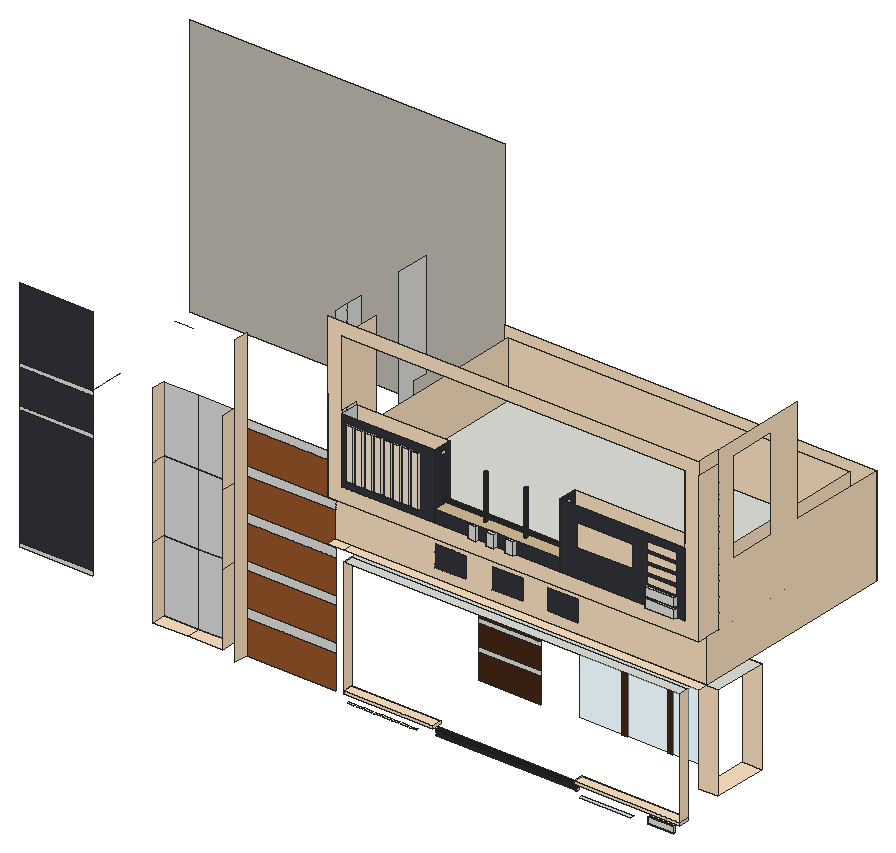
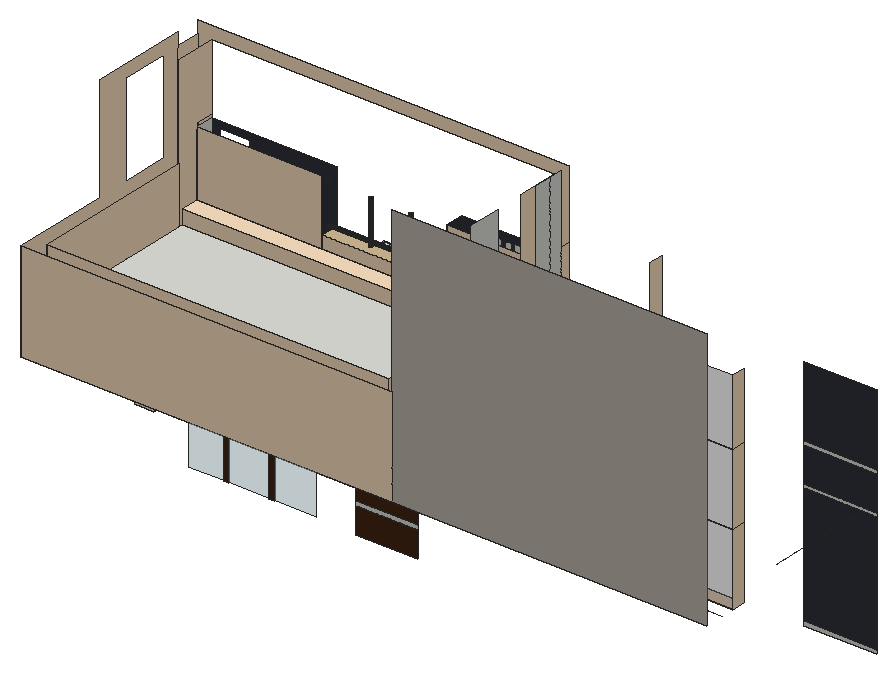
# SketchUp Ruby script. Lengths in inches.
U = 1.inch
M = Sketchup.active_model
def pt(a) = Geom::Point3d.new(a.map { |v| v * U })
def face(e, loops, mat)
  f = e.add_face(loops[0].map { |a| pt(a) })
  loops[1..].each { |l| e.add_face(l.map { |a| pt(a) }).erase! }
  f.material = f.back_material = mat if mat
  f
end
# faces: each face lists its corners as indices into pts; further lists are holes
def faces(e, pts, list, mat = nil) = list.each { |f| face(e, (f[0].is_a?(Array) ? f : [f]).map { |l| l.map { |i| pts[i] } }, mat) }
# xy, xz, yz: faces in a plane at the given z, y or x. An outline is a flat list of corners, or four numbers for a rectangle; further outlines are holes
def ring(l) = l.size == 4 ? [[l[0], l[1]], [l[2], l[1]], [l[2], l[3]], [l[0], l[3]]] : l.each_slice(2).to_a
def flat(e, list, mat, &to3) = list.each { |f| face(e, (f[0].is_a?(Array) ? f : [f]).map { |l| ring(l).map { |u, v| to3.(u, v) } }, mat) }
def xy(e, z, list, mat = nil) = flat(e, list, mat) { |x, y| [x, y, z] }
def xz(e, y, list, mat = nil) = flat(e, list, mat) { |x, z| [x, y, z] }
def yz(e, x, list, mat = nil) = flat(e, list, mat) { |y, z| [x, y, z] }
def lines(e, pts, list) = list.each { |a, b| e.add_line(pt(pts[a]), pt(pts[b])) }
# prism: a flat outline (further loops are holes) pulled along v
def prism(e, loops, v, mat = nil)
  f = face(e, loops, mat); d = Geom::Vector3d.new(v.map { |x| x * U })
  f.pushpull(f.normal.samedirection?(d) ? d.length : -d.length)
end
def box(e, o, s, mat = nil) = prism(e, [[o, [o[0] + s[0], o[1], o[2]], [o[0] + s[0], o[1] + s[1], o[2]], [o[0], o[1] + s[1], o[2]]]], [0, 0, s[2]], mat)
def at(x, y, z, deg = 0) = Geom::Transformation.translation(pt([x, y, z])) * Geom::Transformation.rotation(ORIGIN, Z_AXIS, deg.degrees)
def axes(o, x, y, z) = Geom::Transformation.new([*x, 0, *y, 0, *z, 0, *pt(o).to_a, 1])
def part(name) = M.definitions.add(name)
# library, detail: a bought-in or finely detailed component or shape, given as its bounding box
def library(name, o, s) = part(name).tap { |d| box(d.entities, o, s) }
def detail(e, o, s) = box(e.add_group.entities, o, s)
def put(e, d, t, mat = nil) = e.add_instance(d, t).tap { |i| i.material = mat if mat }
def group(e, t, mat = nil) = e.add_group.tap { |g| g.transformation = t; g.material = mat if mat }.entities
root = M.entities
M.materials.add("[0012_Bisque]").color = [255, 228, 196]
M.materials.add("[0028_AntiqueWhite]").color = [250, 235, 215]
M.materials.add("[Color M08]").color = [30, 30, 30]
M.materials.add("[Color M09]").color = [0, 0, 0]
M.materials.add("[Field Rectangle Tile]").color = [196, 189, 179]
M.materials.add("[Formica Beige]").color = [211, 187, 149]
M.materials.add("[Formica Laminate Dark]").color = [50, 53, 60]
M.materials.add("[Translucent Glass Gray]").color = [128, 128, 128]
M.materials["[Translucent Glass Gray]"].alpha = 0.5
M.materials.add("[Translucent Glass Safety]").color = [204, 235, 244]
M.materials["[Translucent Glass Safety]"].alpha = 0.5
M.materials.add("[Wood Cherry Original]").color = [152, 86, 42]
M.materials.add("[Wood Veneer 01]").color = [68, 40, 21]
box(root,[409.26,39.8,166.78],[15.5,0.87,3.19])
xy(root,166.28,[[409.2,39.8,424.7,40.67]])
xy(root,166.58,[[368.61,38.8,399.74,40.67]])
xy(root,168.02,[[227.93,39.48,232.05,40.67],[233.37,39.48,237.49,40.67],[238.43,39.48,242.55,40.67],[244.05,39.48,248.18,40.67],[249.43,39.48,253.55,40.67],
  [254.74,39.48,258.87,40.67],[260.12,39.48,264.24,40.67],[265.49,39.48,269.62,40.67]],"[0028_AntiqueWhite]")
xy(root,168.7,[[[278.51,42.95,363.63,45.58],[336.54,43.14,336.79,43.17,337.04,43.27,337.24,43.43,337.4,43.64,337.5,43.88,337.54,44.14,337.5,44.4,337.4,44.64,337.24,44.85,337.04,45.01,336.79,45.11,336.54,45.14,336.28,45.11,336.04,45.01,335.83,44.85,335.67,44.64,335.57,44.4,335.54,44.14,335.57,43.88,335.67,43.64,335.83,43.43,336.04,43.27,336.28,43.17]]],"[Color M08]")
xy(root,168.8125,[[305.54,43.14,305.79,43.17,306.04,43.27,306.24,43.43,306.4,43.64,306.5,43.88,306.54,44.14,306.5,44.4,306.4,44.64,306.24,44.85,306.04,45.01,305.79,45.11,305.54,45.14,305.28,45.11,305.04,45.01,304.83,44.85,304.67,44.64,304.57,44.4,304.54,44.14,304.57,43.88,304.67,43.64,304.83,43.43,305.04,43.27,305.28,43.17]])
xy(root,170.07,[[278.51,42.95,363.63,45.58]],"[Color M08]")
xy(root,171.14,[[111.55,38.36,132.61,46.73],[132.61,38.36,153.67,46.73]],"[0012_Bisque]")
xy(root,171.25,[[224.52,40.67,278.51,46.73],[363.63,40.67,427.75,46.73]])
xy(root,173,[[224.52,40.67,278.51,46.73],[363.63,40.67,427.75,46.73]],"[0012_Bisque]")
xy(root,185.0625,[[427.75,54.79,439.21,87.8]],"[0012_Bisque]")
xy(root,242.43,[[224.52,40.67,427.75,46.73],[224.52,46.73,427.75,54.79],[427.75,54.79,439.21,87.8]])
xy(root,249,[[215,46.73,215,162.99,224.52,162.99,224.52,54.79,427.75,54.79,427.75,63.87,439.21,63.87,439.21,46.73],[224.52,54.79,427.75,96.17],[427.75,63.87,439.21,96.36],[224.52,96.17,427.75,107.95],[427.75,96.36,439.21,105.43],
  [427.75,105.43,439.21,174.44],[224.52,107.95,427.75,162.99],[215,162.99,224.52,174.44],[224.52,162.99,427.75,174.44]])
xy(root,249,[[215,40.67,224.52,46.73],[224.52,40.67,439.21,46.73]],"[0012_Bisque]")
xy(root,274.6875,[[215,40.67,223.75,46.73],[223.75,40.67,430.46,46.73],[430.46,40.67,439.21,46.73],[215,46.73,223.75,55.48],[223.75,46.73,430.46,55.48],
  [430.46,46.73,439.21,55.48],[215,55.48,223.75,65.9],[223.75,63.28,430.46,165.7],[215,94.79,223.75,105.21]])
xy(root,283.0625,[[301.05,38.8,305.76,40.67],[312.17,38.8,316.88,40.67],[323.67,38.8,328.38,40.67],[407.7,39.05,425.58,40.67],[223.75,40.67,279.65,51.97],
  [279.65,40.67,355.06,51.97],[355.06,40.67,430.46,51.97]])
xy(root,283.0625,[[223.75,51.97,430.46,63.28]],"[0012_Bisque]")
xy(root,287.67,[[227.14,39.36,231.39,40.67],[232.64,39.36,236.89,40.67],[238.51,39.36,242.76,40.67],[244.08,39.36,248.33,40.67],[249.76,39.36,254.01,40.67],
  [255.33,39.36,259.58,40.67],[260.95,39.36,265.2,40.67],[266.39,39.36,270.64,40.67]])
xy(root,288.0625,[[407.7,39.05,425.58,40.67]])
xy(root,289.37,[[407.7,39.05,425.58,40.67]])
xy(root,290.6875,[[301.05,38.8,305.76,40.67],[312.17,38.8,316.88,40.67],[323.67,38.8,328.38,40.67],[305.63,45.65,305.4,45.68,305.19,45.77,305.01,45.91,304.87,46.09,304.78,46.3,304.75,46.53,304.78,46.75,304.87,46.96,305.01,47.15,305.19,47.29,305.4,47.37,305.63,47.4,305.85,47.37,306.07,47.29,306.25,47.15,306.39,46.96,306.47,46.75,306.5,46.53,306.47,46.3,306.39,46.09,306.25,45.91,306.07,45.77,305.85,45.68],[330.07,45.65,329.84,45.68,329.63,45.77,329.45,45.91,329.31,46.09,329.22,46.3,329.19,46.53,329.22,46.75,329.31,46.96,329.45,47.15,329.63,47.29,329.84,47.37,330.07,47.4,330.29,47.37,330.5,47.29,330.68,47.15,330.82,46.96,330.91,46.75,330.94,46.53,330.91,46.3,330.82,46.09,330.68,45.91,330.5,45.77,330.29,45.68]])
xy(root,290.6875,[[[279.65,40.67,355.06,51.97],[330.07,45.65,329.84,45.68,329.63,45.77,329.45,45.91,329.31,46.09,329.22,46.3,329.19,46.53,329.22,46.75,329.31,46.96,329.45,47.15,329.63,47.29,329.84,47.37,330.07,47.4,330.29,47.37,330.5,47.29,330.68,47.15,330.82,46.96,330.91,46.75,330.94,46.53,330.91,46.3,330.82,46.09,330.68,45.91,330.5,45.77,330.29,45.68],[305.63,45.65,305.4,45.68,305.19,45.77,305.01,45.91,304.87,46.09,304.78,46.3,304.75,46.53,304.78,46.75,304.87,46.96,305.01,47.15,305.19,47.29,305.4,47.37,305.63,47.4,305.85,47.37,306.07,47.29,306.25,47.15,306.39,46.96,306.47,46.75,306.5,46.53,306.47,46.3,306.39,46.09,306.25,45.91,306.07,45.77,305.85,45.68]]],"[Formica Beige]")
xy(root,294.37,[[407.7,39.05,425.58,40.67]])
xz(root,38.8,[[301.05,283.0625,305.76,290.6875],[312.17,283.0625,316.88,290.6875],[323.67,283.0625,328.38,290.6875]])
xz(root,39.05,[[407.7,283.0625,425.58,288.0625],[407.7,289.37,425.58,294.37]])
xz(root,39.36,[[227.14,287.67,231.39,317.98],[232.64,287.67,236.89,317.98],[238.51,287.67,242.76,317.98],[244.08,287.67,248.33,317.98],[249.76,287.67,254.01,317.98],
  [255.33,287.67,259.58,317.98],[260.95,287.67,265.2,317.98],[266.39,287.67,270.64,317.98]],"[0028_AntiqueWhite]")
xz(root,40.67,[[301.05,283.0625,305.76,290.6875],[312.17,283.0625,316.88,290.6875],[323.67,283.0625,328.38,290.6875],[407.7,283.0625,425.58,288.0625],[227.14,287.67,231.39,317.98],
  [232.64,287.67,236.89,317.98],[238.51,287.67,242.76,317.98],[244.08,287.67,248.33,317.98],[249.76,287.67,254.01,317.98],[255.33,287.67,259.58,317.98],
  [260.95,287.67,265.2,317.98],[266.39,287.67,270.64,317.98],[407.7,289.37,425.58,294.37]])
xz(root,40.67,[[224.52,171.25,278.51,173],[363.63,171.25,427.75,173],[215,274.6875,439.21,274.6875,439.21,364.53,430.46,364.53,430.46,283.0625,223.75,283.0625,223.75,364.53,439.21,364.53,439.21,372.25,215,372.25]],"[0012_Bisque]")
xz(root,40.67,[[[223.75,283.0625,279.65,322.3125],[227.14,287.67,231.39,317.98],[232.64,287.67,236.89,317.98],[238.51,287.67,242.76,317.98],[244.08,287.67,248.33,317.98],[249.76,287.67,254.01,317.98],[255.33,287.67,259.58,317.98],[260.95,287.67,265.2,317.98],[266.39,287.67,270.64,317.98]],[279.65,283.0625,301.05,290.6875],[305.76,283.0625,312.17,290.6875],[316.88,283.0625,323.67,290.6875],[328.38,283.0625,355.06,290.6875],
  [[355.06,283.0625,407.7,283.0625,407.7,288.0625,425.58,288.0625,425.58,283.0625,430.46,283.0625,430.46,322.3125,355.06,322.3125],[365.58,300,398.96,313.68],[407.7,313.43,425.58,318.43],[407.7,307.12,425.58,312.12],[407.7,301.12,425.58,306.12],[407.7,294.93,425.58,299.93],[407.7,289.37,425.58,294.37]]],"[Formica Laminate Dark]")
xz(root,42.95,[[278.51,168.7,363.63,170.07]],"[Color M08]")
xz(root,45.58,[[278.51,168.7,363.63,170.07]],"[Color M08]")
xz(root,46.73,[[24.6875,177.73,68.38,180.02],[161.14,187.61,215,192.76],[161.14,213.23,215,218.39],[161.14,238.86,215,244.01],[24.6875,251.85,68.38,254.15],
  [161.14,264.48,215,269.64],[24.6875,275.16,68.38,277.46],[161.14,290.11,215,295.26]])
xz(root,46.73,[[224.52,171.25,278.51,173],[363.63,171.25,427.75,173],[[215,249,439.21,274.6875],[275.14,254.7,294.2,267.83],[309.26,254.7,328.33,267.83],[342.45,254.7,361.51,267.83]]],"[0012_Bisque]")
xz(root,46.73,[[24.6875,180.02,68.38,251.85],[24.6875,254.15,68.38,275.16],[275.14,254.7,294.2,267.83],[309.26,254.7,328.33,267.83],[342.45,254.7,361.51,267.83],
  [24.6875,277.46,68.38,320.49]],"[Formica Laminate Dark]")
xz(root,46.73,[[111.55,171.14,132.61,214.3125],[132.61,171.14,153.67,214.3125],[111.55,214.3125,132.61,257.49],[132.61,214.3125,153.67,257.49],[111.55,257.49,132.61,297.86],
  [132.61,257.49,153.67,297.86]],"[Translucent Glass Gray]")
xz(root,46.73,[[161.14,167.14,215,187.61],[161.14,192.76,215,213.23],[161.14,218.39,215,238.86],[161.14,244.01,215,264.48],[161.14,269.64,215,290.11]],"[Wood Cherry Original]")
xz(root,51.97,[[223.75,283.0625,279.65,322.3125],[279.65,283.0625,355.06,290.6875],[355.06,283.0625,430.46,322.3125]],"[0012_Bisque]")
xz(root,54.79,[[224.52,242.43,427.75,249],[224.52,249,228.84,256],[228.84,249,427.75,256]])
xz(root,54.79,[[427.75,185.0625,439.21,242.43]],"[0012_Bisque]")
xz(root,63.28,[[223.75,274.6875,430.46,283.0625]],"[0012_Bisque]")
xz(root,65.9,[[215,274.6875,223.75,308.625]])
xz(root,87.8,[[427.75,185.0625,439.21,242.43]],"[0012_Bisque]")
xz(root,96.17,[[262.03,183.03,299.47,185.625],[262.03,198.54,299.47,201.14],[262.03,213.04,299.47,215.64]])
xz(root,96.17,[[323.03,168.34,348.35,229.59],[351.56,168.34,375.78,229.59],[379,168.34,399.97,229.59]],"[Translucent Glass Safety]")
xz(root,96.17,[[262.03,167.51,299.47,183.03],[348.35,168.34,351.56,229.59],[375.78,168.34,379,229.59],[262.03,185.625,299.47,198.54],[262.03,201.14,299.47,213.04],
  [262.03,215.64,299.47,230.51]],"[Wood Veneer 01]")
xz(root,165.7,[[223.75,274.6875,430.46,308.625]],"[0012_Bisque]")
xz(root,174.44,[[215,249,439.21,308.625]],"[0012_Bisque]")
xz(root,174.44,[[24.6875,249,215,406.75]],"[Field Rectangle Tile]")
yz(root,111.55,[[38.36,171.14,46.73,214.3125],[38.36,214.3125,46.73,257.49],[38.36,257.49,46.73,297.86]],"[0012_Bisque]")
yz(root,153.67,[[38.36,171.14,46.73,214.3125],[38.36,214.3125,46.73,257.49],[38.36,257.49,46.73,297.86]],"[0012_Bisque]")
yz(root,161.14,[[38.36,167.14,46.73,341.36]],"[0012_Bisque]")
yz(root,215,[[46.73,274.6875,55.48,372.25],[55.48,274.6875,65.9,372.25],[94.79,274.6875,105.21,274.6875,105.21,308.625,114.71,308.625,114.71,372.25,94.79,372.25]])
yz(root,215,[[40.67,274.6875,46.73,330.3125]],"[0012_Bisque]")
yz(root,223.75,[[40.67,283.0625,51.97,322.3125]])
yz(root,223.75,[[63.28,274.6875,65.9,274.6875,65.9,364.53,40.67,364.53,40.67,324.5,51.97,324.5,51.97,283.0625,63.28,283.0625],[65.9,274.6875,165.7,308.625]],"[0012_Bisque]")
yz(root,224.52,[[40.67,171.25,46.73,173]])
yz(root,224.52,[[40.67,173,46.73,242.43]],"[0012_Bisque]")
yz(root,227.14,[[39.36,287.67,40.67,317.98]],"[0028_AntiqueWhite]")
yz(root,231.39,[[39.36,287.67,40.67,317.98]],"[0028_AntiqueWhite]")
yz(root,232.64,[[39.36,287.67,40.67,317.98]],"[0028_AntiqueWhite]")
yz(root,236.89,[[39.36,287.67,40.67,317.98]],"[0028_AntiqueWhite]")
yz(root,238.51,[[39.36,287.67,40.67,317.98]],"[0028_AntiqueWhite]")
yz(root,242.76,[[39.36,287.67,40.67,317.98]],"[0028_AntiqueWhite]")
yz(root,244.08,[[39.36,287.67,40.67,317.98]],"[0028_AntiqueWhite]")
yz(root,248.33,[[39.36,287.67,40.67,317.98]],"[0028_AntiqueWhite]")
yz(root,249.76,[[39.36,287.67,40.67,317.98]],"[0028_AntiqueWhite]")
yz(root,254.01,[[39.36,287.67,40.67,317.98]],"[0028_AntiqueWhite]")
yz(root,255.33,[[39.36,287.67,40.67,317.98]],"[0028_AntiqueWhite]")
yz(root,259.58,[[39.36,287.67,40.67,317.98]],"[0028_AntiqueWhite]")
yz(root,260.95,[[39.36,287.67,40.67,317.98]],"[0028_AntiqueWhite]")
yz(root,265.2,[[39.36,287.67,40.67,317.98]],"[0028_AntiqueWhite]")
yz(root,266.39,[[39.36,287.67,40.67,317.98]],"[0028_AntiqueWhite]")
yz(root,270.64,[[39.36,287.67,40.67,317.98]],"[0028_AntiqueWhite]")
yz(root,278.51,[[40.67,171.25,46.73,173]],"[0012_Bisque]")
yz(root,279.65,[[40.67,283.0625,51.97,290.6875],[46.99,292.52,46.77,292.55,46.55,292.64,46.375,292.78,46.23,292.96,46.15,293.17,46.12,293.4,46.15,293.625,46.23,293.84,46.375,294.02,46.55,294.16,46.77,294.24,46.99,294.27,47.22,294.24,47.43,294.16,47.61,294.02,47.75,293.84,47.84,293.625,47.87,293.4,47.84,293.17,47.75,292.96,47.61,292.78,47.43,292.64,47.22,292.55]])
yz(root,279.65,[[[40.67,290.6875,51.97,322.3125],[45.65,317.125,49.39,319.4375],[46.99,313.02,46.77,313.05,46.55,313.14,46.375,313.28,46.23,313.46,46.15,313.67,46.12,313.9,46.15,314.125,46.23,314.34,46.375,314.52,46.55,314.66,46.77,314.74,46.99,314.77,47.22,314.74,47.43,314.66,47.61,314.52,47.75,314.34,47.84,314.125,47.87,313.9,47.84,313.67,47.75,313.46,47.61,313.28,47.43,313.14,47.22,313.05],[46.99,292.52,46.77,292.55,46.55,292.64,46.375,292.78,46.23,292.96,46.15,293.17,46.12,293.4,46.15,293.625,46.23,293.84,46.375,294.02,46.55,294.16,46.77,294.24,46.99,294.27,47.22,294.24,47.43,294.16,47.61,294.02,47.75,293.84,47.84,293.625,47.87,293.4,47.84,293.17,47.75,292.96,47.61,292.78,47.43,292.64,47.22,292.55],[46.99,308.96,46.77,308.99,46.55,309.08,46.375,309.22,46.23,309.4,46.15,309.61,46.12,309.84,46.15,310.0625,46.23,310.27,46.375,310.45,46.55,310.59,46.77,310.68,46.99,310.71,47.22,310.68,47.43,310.59,47.61,310.45,47.75,310.27,47.84,310.0625,47.87,309.84,47.84,309.61,47.75,309.4,47.61,309.22,47.43,309.08,47.22,308.99],[46.99,296.71,46.77,296.74,46.55,296.83,46.375,296.97,46.23,297.15,46.15,297.36,46.12,297.59,46.15,297.8125,46.23,298.02,46.375,298.2,46.55,298.34,46.77,298.43,46.99,298.46,47.22,298.43,47.43,298.34,47.61,298.2,47.75,298.02,47.84,297.8125,47.87,297.59,47.84,297.36,47.75,297.15,47.61,296.97,47.43,296.83,47.22,296.74],[46.99,305.27,46.77,305.3,46.55,305.39,46.375,305.53,46.23,305.71,46.15,305.92,46.12,306.15,46.15,306.375,46.23,306.59,46.375,306.77,46.55,306.91,46.77,306.99,46.99,307.02,47.22,306.99,47.43,306.91,47.61,306.77,47.75,306.59,47.84,306.375,47.87,306.15,47.84,305.92,47.75,305.71,47.61,305.53,47.43,305.39,47.22,305.3],[46.99,300.84,46.77,300.87,46.55,300.95,46.375,301.09,46.23,301.27,46.15,301.48,46.12,301.71,46.15,301.9375,46.23,302.15,46.375,302.33,46.55,302.47,46.77,302.56,46.99,302.59,47.22,302.56,47.43,302.47,47.61,302.33,47.75,302.15,47.84,301.9375,47.87,301.71,47.84,301.48,47.75,301.27,47.61,301.09,47.43,300.95,47.22,300.87]]],"[Formica Laminate Dark]")
yz(root,301.05,[[38.8,283.0625,40.67,290.6875]])
yz(root,305.76,[[38.8,283.0625,40.67,290.6875]])
yz(root,312.17,[[38.8,283.0625,40.67,290.6875]])
yz(root,316.88,[[38.8,283.0625,40.67,290.6875]])
yz(root,323.67,[[38.8,283.0625,40.67,290.6875]])
yz(root,328.38,[[38.8,283.0625,40.67,290.6875]])
yz(root,355.06,[[40.67,283.0625,51.97,290.6875]])
yz(root,355.06,[[[40.67,290.6875,51.97,322.3125],[45.65,317.125,49.39,319.4375],[46.99,313.02,47.22,313.05,47.43,313.14,47.61,313.28,47.75,313.46,47.84,313.67,47.87,313.9,47.84,314.125,47.75,314.34,47.61,314.52,47.43,314.66,47.22,314.74,46.99,314.77,46.77,314.74,46.55,314.66,46.375,314.52,46.23,314.34,46.15,314.125,46.12,313.9,46.15,313.67,46.23,313.46,46.375,313.28,46.55,313.14,46.77,313.05],[46.99,308.96,47.22,308.99,47.43,309.08,47.61,309.22,47.75,309.4,47.84,309.61,47.87,309.84,47.84,310.0625,47.75,310.27,47.61,310.45,47.43,310.59,47.22,310.68,46.99,310.71,46.77,310.68,46.55,310.59,46.375,310.45,46.23,310.27,46.15,310.0625,46.12,309.84,46.15,309.61,46.23,309.4,46.375,309.22,46.55,309.08,46.77,308.99],[46.99,305.27,47.22,305.3,47.43,305.39,47.61,305.53,47.75,305.71,47.84,305.92,47.87,306.15,47.84,306.375,47.75,306.59,47.61,306.77,47.43,306.91,47.22,306.99,46.99,307.02,46.77,306.99,46.55,306.91,46.375,306.77,46.23,306.59,46.15,306.375,46.12,306.15,46.15,305.92,46.23,305.71,46.375,305.53,46.55,305.39,46.77,305.3],[46.99,300.84,47.22,300.87,47.43,300.95,47.61,301.09,47.75,301.27,47.84,301.48,47.87,301.71,47.84,301.9375,47.75,302.15,47.61,302.33,47.43,302.47,47.22,302.56,46.99,302.59,46.77,302.56,46.55,302.47,46.375,302.33,46.23,302.15,46.15,301.9375,46.12,301.71,46.15,301.48,46.23,301.27,46.375,301.09,46.55,300.95,46.77,300.87],[46.99,296.71,47.22,296.74,47.43,296.83,47.61,296.97,47.75,297.15,47.84,297.36,47.87,297.59,47.84,297.8125,47.75,298.02,47.61,298.2,47.43,298.34,47.22,298.43,46.99,298.46,46.77,298.43,46.55,298.34,46.375,298.2,46.23,298.02,46.15,297.8125,46.12,297.59,46.15,297.36,46.23,297.15,46.375,296.97,46.55,296.83,46.77,296.74],[46.99,292.52,47.22,292.55,47.43,292.64,47.61,292.78,47.75,292.96,47.84,293.17,47.87,293.4,47.84,293.625,47.75,293.84,47.61,294.02,47.43,294.16,47.22,294.24,46.99,294.27,46.77,294.24,46.55,294.16,46.375,294.02,46.23,293.84,46.15,293.625,46.12,293.4,46.15,293.17,46.23,292.96,46.375,292.78,46.55,292.64,46.77,292.55]]],"[Formica Laminate Dark]")
yz(root,363.63,[[43.9,166.34,44.06,166.36,44.22,166.42,44.35,166.51,44.45,166.64,44.52,166.79,44.55,166.95,44.53,167.11,44.47,167.26,44.38,167.4,44.25,167.5,44.11,167.57,43.94,167.59,43.78,167.58,43.63,167.52,43.5,167.43,43.39,167.3,43.33,167.15,43.3,166.99,43.3125,166.83,43.37,166.68,43.47,166.54,43.59,166.4375,43.74,166.37],[42.95,168.7,45.58,170.07]])
yz(root,363.63,[[40.67,171.25,46.73,173]],"[0012_Bisque]")
yz(root,407.7,[[39.05,283.0625,40.67,288.0625],[39.05,289.37,40.67,294.37]])
yz(root,425.58,[[39.05,283.0625,40.67,288.0625],[39.05,289.37,40.67,294.37]])
yz(root,427.75,[[40.67,171.25,46.73,173]])
yz(root,427.75,[[40.67,173,46.73,242.43]],"[0012_Bisque]")
yz(root,430.46,[[40.67,283.0625,51.97,322.3125]])
yz(root,430.46,[[63.28,274.6875,63.28,283.0625,51.97,283.0625,51.97,324.5,40.67,324.5,40.67,364.53,65.9,364.53,65.9,274.6875],[65.9,274.6875,165.7,308.625]],"[0012_Bisque]")
yz(root,439.21,[[[46.73,249,174.44,249,174.44,308.625,114.71,308.625,114.71,372.25,55.48,372.25,55.48,274.6875,46.73,274.6875],[65.9,308.625,94.79,364.53]],[40.67,274.6875,55.48,364.53]],"[0012_Bisque]")
p = [[363.63,43.9,166.34],[363.63,43.74,166.37],[278.51,43.74,166.37],[278.51,43.9,166.34],[363.63,44.06,166.36],[278.51,44.06,166.36],
  [363.63,43.59,166.4375],[363.63,43.47,166.54],[278.51,43.47,166.54],[278.51,43.59,166.4375],[363.63,44.22,166.42],[278.51,44.22,166.42],
  [363.63,44.35,166.51],[278.51,44.35,166.51],[363.63,43.37,166.68],[278.51,43.37,166.68],[363.63,44.45,166.64],[278.51,44.45,166.64],
  [363.63,44.52,166.79],[278.51,44.52,166.79],[363.63,43.3125,166.83],[278.51,43.3125,166.83],[363.63,43.3,166.99],[278.51,43.3,166.99],
  [363.63,44.55,166.95],[278.51,44.55,166.95],[363.63,44.53,167.11],[278.51,44.53,167.11],[363.63,43.33,167.15],[278.51,43.33,167.15],
  [363.63,44.47,167.26],[278.51,44.47,167.26],[363.63,43.39,167.3],[278.51,43.39,167.3],[363.63,43.5,167.43],[278.51,43.5,167.43],
  [363.63,44.38,167.4],[278.51,44.38,167.4],[363.63,43.63,167.52],[278.51,43.63,167.52],[363.63,44.25,167.5],[278.51,44.25,167.5],
  [363.63,43.78,167.58],[278.51,43.78,167.58],[363.63,44.11,167.57],[278.51,44.11,167.57],[363.63,43.94,167.59],[278.51,43.94,167.59],
  [305.19,45.77,290.6875],[305.4,45.68,290.6875],[305.4,45.68,317.125],[305.19,45.77,317.125],[305.63,45.65,290.6875],[305.63,45.65,317.125],
  [305.85,45.68,290.6875],[305.85,45.68,317.125],[306.07,45.77,290.6875],[306.07,45.77,317.125],[329.63,45.77,290.6875],[329.84,45.68,290.6875],
  [329.84,45.68,317.125],[329.63,45.77,317.125],[330.07,45.65,290.6875],[330.07,45.65,317.125],[330.29,45.68,290.6875],[330.29,45.68,317.125],
  [330.5,45.77,290.6875],[330.5,45.77,317.125],[305.01,45.91,290.6875],[305.01,45.91,317.125],[306.25,45.91,290.6875],[306.25,45.91,317.125],
  [329.45,45.91,290.6875],[329.45,45.91,317.125],[330.68,45.91,290.6875],[330.68,45.91,317.125],[304.87,46.09,290.6875],[304.87,46.09,317.125],
  [306.39,46.09,290.6875],[306.39,46.09,317.125],[329.31,46.09,290.6875],[329.31,46.09,317.125],[330.82,46.09,290.6875],[330.82,46.09,317.125],
  [304.78,46.3,290.6875],[304.78,46.3,317.125],[306.47,46.3,290.6875],[306.47,46.3,317.125],[329.22,46.3,290.6875],[329.22,46.3,317.125],
  [330.91,46.3,290.6875],[330.91,46.3,317.125],[304.75,46.53,290.6875],[304.75,46.53,317.125],[306.5,46.53,290.6875],[306.5,46.53,317.125],
  [329.19,46.53,290.6875],[329.19,46.53,317.125],[330.94,46.53,290.6875],[330.94,46.53,317.125],[304.78,46.75,290.6875],[304.78,46.75,317.125],
  [306.47,46.75,290.6875],[306.47,46.75,317.125],[329.22,46.75,290.6875],[329.22,46.75,317.125],[330.91,46.75,290.6875],[330.91,46.75,317.125],
  [304.87,46.96,290.6875],[304.87,46.96,317.125],[306.39,46.96,290.6875],[306.39,46.96,317.125],[329.31,46.96,290.6875],[329.31,46.96,317.125],
  [330.82,46.96,290.6875],[330.82,46.96,317.125],[305.01,47.15,290.6875],[305.01,47.15,317.125],[306.25,47.15,290.6875],[306.25,47.15,317.125],
  [329.45,47.15,290.6875],[329.45,47.15,317.125],[330.68,47.15,290.6875],[330.68,47.15,317.125],[305.19,47.29,290.6875],[305.19,47.29,317.125],
  [306.07,47.29,290.6875],[306.07,47.29,317.125],[329.63,47.29,290.6875],[329.63,47.29,317.125],[330.5,47.29,290.6875],[330.5,47.29,317.125],
  [305.4,47.37,290.6875],[305.4,47.37,317.125],[305.85,47.37,290.6875],[305.85,47.37,317.125],[329.84,47.37,290.6875],[329.84,47.37,317.125],
  [330.29,47.37,290.6875],[330.29,47.37,317.125],[305.63,47.4,290.6875],[305.63,47.4,317.125],[330.07,47.4,290.6875],[330.07,47.4,317.125],
  [279.65,46.77,292.55],[279.65,46.99,292.52],[355.06,46.99,292.52],[355.06,46.77,292.55],[279.65,47.22,292.55],[355.06,47.22,292.55],
  [279.65,46.375,292.78],[279.65,46.55,292.64],[355.06,46.55,292.64],[355.06,46.375,292.78],[279.65,47.43,292.64],[355.06,47.43,292.64],
  [279.65,47.61,292.78],[355.06,47.61,292.78],[279.65,46.23,292.96],[355.06,46.23,292.96],[279.65,47.75,292.96],[355.06,47.75,292.96],
  [279.65,46.15,293.17],[355.06,46.15,293.17],[279.65,47.84,293.17],[355.06,47.84,293.17],[279.65,46.12,293.4],[355.06,46.12,293.4],
  [279.65,47.87,293.4],[355.06,47.87,293.4],[279.65,46.15,293.625],[355.06,46.15,293.625],[279.65,47.84,293.625],[355.06,47.84,293.625],
  [279.65,46.23,293.84],[355.06,46.23,293.84],[279.65,47.75,293.84],[355.06,47.75,293.84],[279.65,46.375,294.02],[355.06,46.375,294.02],
  [279.65,47.61,294.02],[355.06,47.61,294.02],[279.65,46.55,294.16],[355.06,46.55,294.16],[279.65,47.43,294.16],[355.06,47.43,294.16],
  [279.65,46.77,294.24],[355.06,46.77,294.24],[279.65,46.99,294.27],[355.06,46.99,294.27],[279.65,47.22,294.24],[355.06,47.22,294.24],
  [36.15,162.99,249],[24.6875,162.99,249],[36.15,107.95,249],[36.15,46.73,249],[228.84,54.79,256],[228.84,162.99,256],
  [427.75,54.79,256],[427.75,162.99,256],[430.46,55.48,274.6875],[430.46,63.28,274.6875],[430.46,65.9,274.6875],[439.21,65.9,274.6875],
  [430.46,105.21,274.6875],[439.21,105.21,274.6875],[439.21,94.79,274.6875],[430.46,94.79,274.6875]]
faces(root,p,[[0,1,2,3],[4,0,3,5],[6,7,8,9],[1,6,9,2],[10,4,5,11],[12,10,11,13],[7,14,15,8],[16,12,13,17],
  [18,16,17,19],[14,20,21,15],[20,22,23,21],[24,18,19,25],[26,24,25,27],[22,28,29,23],[30,26,27,31],[28,32,33,29],
  [32,34,35,33],[36,30,31,37],[34,38,39,35],[40,36,37,41],[38,42,43,39],[44,40,41,45],[42,46,47,43],[46,44,45,47]],"[Color M08]")
faces(root,p,[[48,49,50,51],[49,52,53,50],[52,54,55,53],[54,56,57,55],[58,59,60,61],[59,62,63,60],[62,64,65,63],[64,66,67,65],
  [68,48,51,69],[56,70,71,57],[72,58,61,73],[66,74,75,67],[76,68,69,77],[70,78,79,71],[80,72,73,81],[74,82,83,75],
  [84,76,77,85],[78,86,87,79],[88,80,81,89],[82,90,91,83],[92,84,85,93],[86,94,95,87],[96,88,89,97],[90,98,99,91],
  [100,92,93,101],[94,102,103,95],[104,96,97,105],[98,106,107,99],[108,100,101,109],[102,110,111,103],[112,104,105,113],[106,114,115,107],
  [116,108,109,117],[110,118,119,111],[120,112,113,121],[114,122,123,115],[124,116,117,125],[118,126,127,119],[128,120,121,129],[122,130,131,123],
  [132,124,125,133],[126,134,135,127],[136,128,129,137],[130,138,139,131],[140,132,133,141],[134,140,141,135],[142,136,137,143],[138,142,143,139],
  [144,145,146,147],[145,148,149,146],[150,151,152,153],[151,144,147,152],[148,154,155,149],[154,156,157,155],[158,150,153,159],[156,160,161,157],
  [162,158,159,163],[160,164,165,161],[166,162,163,167],[164,168,169,165],[170,166,167,171],[168,172,173,169],[174,170,171,175],[172,176,177,173],
  [178,174,175,179],[176,180,181,177],[182,178,179,183],[180,184,185,181],[186,182,183,187],[188,186,187,189],[190,188,189,191],[184,190,191,185]],"[Color M09]")
lines(root,p,[[192,193],[194,195],[196,197],[198,199],[200,201],[202,203],[204,205],[206,207]])
